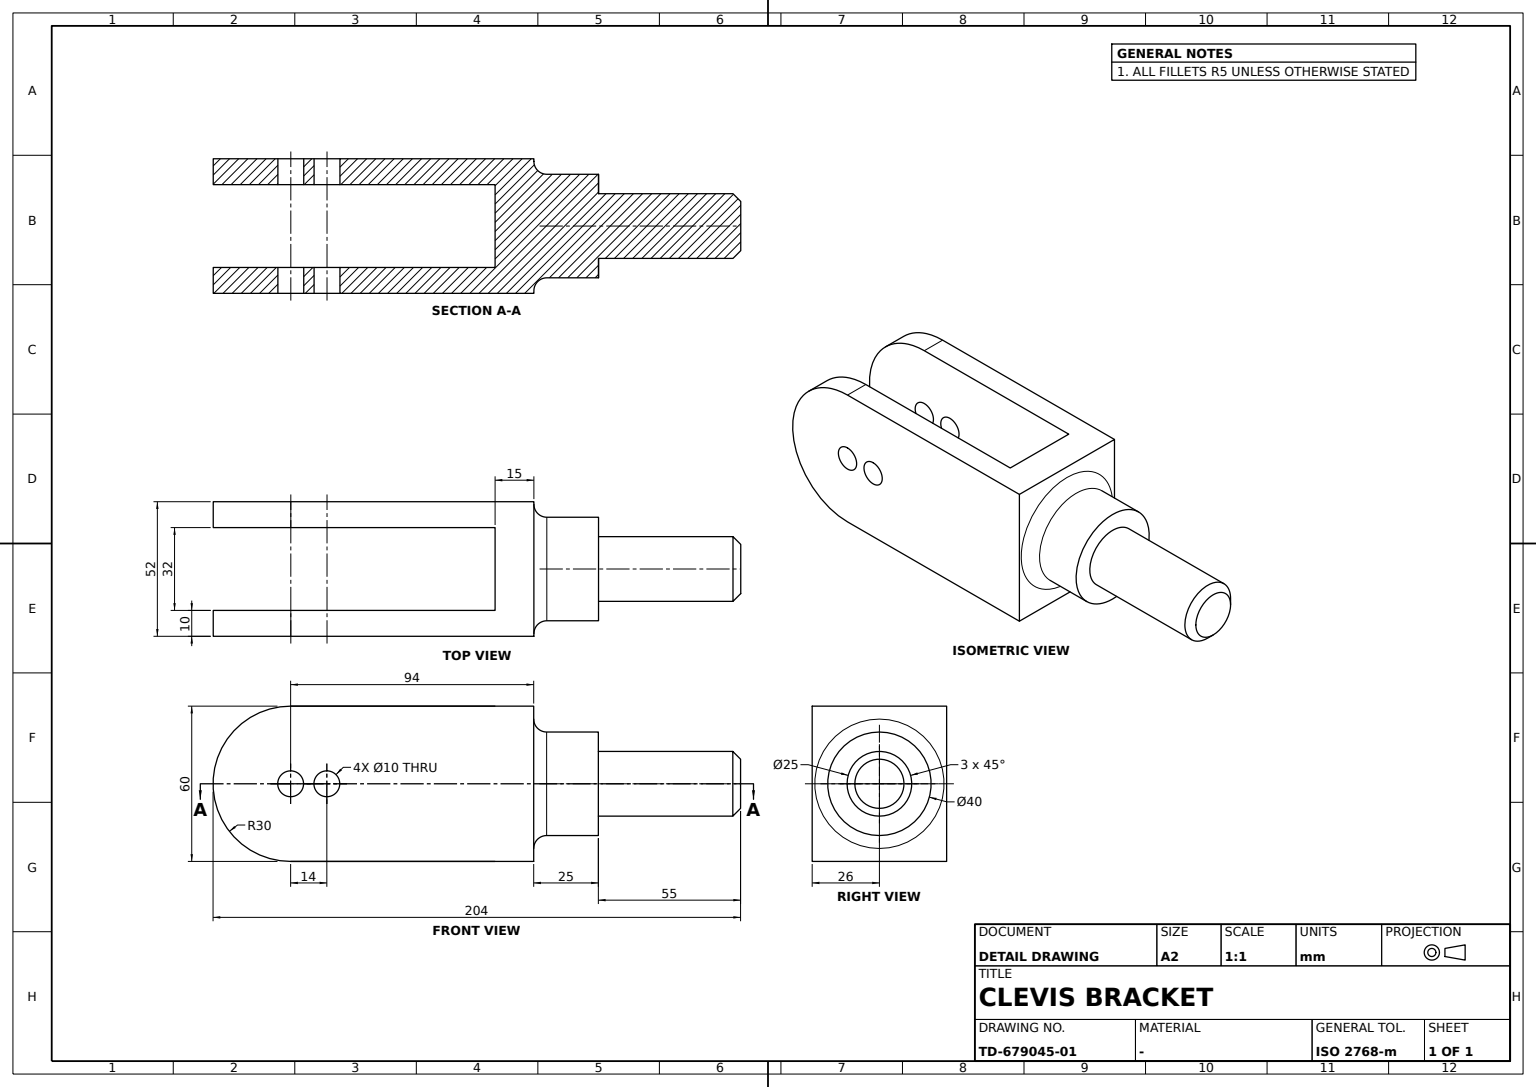
ISO-10303-21;
HEADER;
FILE_DESCRIPTION((''),'2;1');
FILE_NAME('','',(''),(''),'','','');
FILE_SCHEMA(('AUTOMOTIVE_DESIGN'));
ENDSEC;
DATA;
#1=APPLICATION_CONTEXT('');
#2=PRODUCT_CONTEXT('',#1,'mechanical');
#3=PRODUCT('','','',(#2));
#4=PRODUCT_DEFINITION_FORMATION('','',#3);
#5=PRODUCT_DEFINITION_CONTEXT('',#1,'design');
#6=PRODUCT_DEFINITION('','',#4,#5);
#7=PRODUCT_DEFINITION_SHAPE('','',#6);
#8=(LENGTH_UNIT()NAMED_UNIT(*)SI_UNIT(.MILLI.,.METRE.));
#9=(NAMED_UNIT(*)PLANE_ANGLE_UNIT()SI_UNIT($,.RADIAN.));
#10=(NAMED_UNIT(*)SI_UNIT($,.STERADIAN.)SOLID_ANGLE_UNIT());
#11=UNCERTAINTY_MEASURE_WITH_UNIT(LENGTH_MEASURE(0.005),#8,'distance_accuracy_value','');
#12=(GEOMETRIC_REPRESENTATION_CONTEXT(3)GLOBAL_UNCERTAINTY_ASSIGNED_CONTEXT((#11))GLOBAL_UNIT_ASSIGNED_CONTEXT((#8,#9,#10))REPRESENTATION_CONTEXT('',''));
#13=CARTESIAN_POINT('',(-94.,10.,5.));
#14=VERTEX_POINT('',#13);
#15=CARTESIAN_POINT('',(-94.,10.,0.));
#16=DIRECTION('',(0.,1.,0.));
#17=DIRECTION('',(0.,0.,1.));
#18=AXIS2_PLACEMENT_3D('',#15,#16,#17);
#19=CIRCLE('',#18,5.);
#20=EDGE_CURVE('',#14,#14,#19,.T.);
#21=ORIENTED_EDGE('',*,*,#20,.T.);
#22=EDGE_LOOP('',(#21));
#23=FACE_BOUND('',#22,.T.);
#24=CARTESIAN_POINT('',(-94.,0.,5.));
#25=VERTEX_POINT('',#24);
#26=CARTESIAN_POINT('',(-94.,0.,0.));
#27=AXIS2_PLACEMENT_3D('',#26,#16,#17);
#28=CIRCLE('',#27,5.);
#29=EDGE_CURVE('',#25,#25,#28,.T.);
#30=ORIENTED_EDGE('',*,*,#29,.F.);
#31=EDGE_LOOP('',(#30));
#32=FACE_BOUND('',#31,.T.);
#33=CARTESIAN_POINT('',(-94.,5.,0.));
#34=DIRECTION('',(-1.,0.,0.));
#35=AXIS2_PLACEMENT_3D('',#33,#16,#34);
#36=CYLINDRICAL_SURFACE('',#35,5.);
#37=ADVANCED_FACE('',(#23,#32),#36,.F.);
#38=CARTESIAN_POINT('',(-15.,10.,30.));
#39=VERTEX_POINT('',#38);
#40=CARTESIAN_POINT('',(-15.,10.,-30.));
#41=VERTEX_POINT('',#40);
#42=CARTESIAN_POINT('',(-15.,10.,0.));
#43=DIRECTION('',(0.,0.,-1.));
#44=VECTOR('',#43,1000.);
#45=LINE('',#42,#44);
#46=EDGE_CURVE('',#39,#41,#45,.T.);
#47=ORIENTED_EDGE('',*,*,#46,.F.);
#48=CARTESIAN_POINT('',(-15.,42.,30.));
#49=VERTEX_POINT('',#48);
#50=VECTOR('',#16,1000.);
#51=LINE('',#38,#50);
#52=EDGE_CURVE('',#39,#49,#51,.T.);
#53=ORIENTED_EDGE('',*,*,#52,.T.);
#54=CARTESIAN_POINT('',(-15.,42.,-30.));
#55=VERTEX_POINT('',#54);
#56=CARTESIAN_POINT('',(-15.,42.,0.));
#57=LINE('',#56,#44);
#58=EDGE_CURVE('',#49,#55,#57,.T.);
#59=ORIENTED_EDGE('',*,*,#58,.T.);
#60=CARTESIAN_POINT('',(-15.,0.,-30.));
#61=LINE('',#60,#50);
#62=EDGE_CURVE('',#41,#55,#61,.T.);
#63=ORIENTED_EDGE('',*,*,#62,.F.);
#64=EDGE_LOOP('',(#47,#53,#59,#63));
#65=FACE_BOUND('',#64,.T.);
#66=DIRECTION('',(1.,0.,0.));
#67=AXIS2_PLACEMENT_3D('',#38,#66,#43);
#68=PLANE('',#67);
#69=ADVANCED_FACE('',(#65),#68,.F.);
#70=CARTESIAN_POINT('',(0.,26.,25.));
#71=VERTEX_POINT('',#70);
#72=CARTESIAN_POINT('',(0.,26.,0.));
#73=AXIS2_PLACEMENT_3D('',#72,#34,#17);
#74=CIRCLE('',#73,25.);
#75=EDGE_CURVE('',#71,#71,#74,.T.);
#76=ORIENTED_EDGE('',*,*,#75,.F.);
#77=EDGE_LOOP('',(#76));
#78=FACE_BOUND('',#77,.T.);
#79=CARTESIAN_POINT('',(5.,26.,-20.));
#80=VERTEX_POINT('',#79);
#81=CARTESIAN_POINT('',(5.,26.,0.));
#82=AXIS2_PLACEMENT_3D('',#81,#66,#43);
#83=CIRCLE('',#82,20.);
#84=EDGE_CURVE('',#80,#80,#83,.F.);
#85=ORIENTED_EDGE('',*,*,#84,.T.);
#86=EDGE_LOOP('',(#85));
#87=FACE_BOUND('',#86,.T.);
#88=DIRECTION('',(0.,-0.5,-0.866025404));
#89=AXIS2_PLACEMENT_3D('',#81,#34,#88);
#90=TOROIDAL_SURFACE('',#89,25.,5.);
#91=ADVANCED_FACE('',(#78,#87),#90,.F.);
#92=CARTESIAN_POINT('',(-80.,42.,5.));
#93=VERTEX_POINT('',#92);
#94=CARTESIAN_POINT('',(-80.,42.,0.));
#95=AXIS2_PLACEMENT_3D('',#94,#16,#17);
#96=CIRCLE('',#95,5.);
#97=EDGE_CURVE('',#93,#93,#96,.T.);
#98=ORIENTED_EDGE('',*,*,#97,.F.);
#99=EDGE_LOOP('',(#98));
#100=FACE_BOUND('',#99,.T.);
#101=CARTESIAN_POINT('',(-80.,52.,5.));
#102=VERTEX_POINT('',#101);
#103=CARTESIAN_POINT('',(-80.,52.,0.));
#104=AXIS2_PLACEMENT_3D('',#103,#16,#17);
#105=CIRCLE('',#104,5.);
#106=EDGE_CURVE('',#102,#102,#105,.T.);
#107=ORIENTED_EDGE('',*,*,#106,.T.);
#108=EDGE_LOOP('',(#107));
#109=FACE_BOUND('',#108,.T.);
#110=CARTESIAN_POINT('',(-80.,5.,0.));
#111=AXIS2_PLACEMENT_3D('',#110,#16,#34);
#112=CYLINDRICAL_SURFACE('',#111,5.);
#113=ADVANCED_FACE('',(#100,#109),#112,.F.);
#114=ORIENTED_EDGE('',*,*,#52,.F.);
#115=CARTESIAN_POINT('',(-94.,10.,30.));
#116=VERTEX_POINT('',#115);
#117=CARTESIAN_POINT('',(0.,10.,30.));
#118=VECTOR('',#34,1000.);
#119=LINE('',#117,#118);
#120=EDGE_CURVE('',#39,#116,#119,.T.);
#121=ORIENTED_EDGE('',*,*,#120,.T.);
#122=CARTESIAN_POINT('',(-94.,0.,30.));
#123=VERTEX_POINT('',#122);
#124=CARTESIAN_POINT('',(-94.,5.,30.));
#125=LINE('',#124,#50);
#126=EDGE_CURVE('',#123,#116,#125,.T.);
#127=ORIENTED_EDGE('',*,*,#126,.F.);
#128=CARTESIAN_POINT('',(0.,0.,30.));
#129=VERTEX_POINT('',#128);
#130=LINE('',#128,#118);
#131=EDGE_CURVE('',#129,#123,#130,.T.);
#132=ORIENTED_EDGE('',*,*,#131,.F.);
#133=CARTESIAN_POINT('',(0.,52.,30.));
#134=VERTEX_POINT('',#133);
#135=LINE('',#128,#50);
#136=EDGE_CURVE('',#129,#134,#135,.T.);
#137=ORIENTED_EDGE('',*,*,#136,.T.);
#138=CARTESIAN_POINT('',(-94.,52.,30.));
#139=VERTEX_POINT('',#138);
#140=LINE('',#133,#118);
#141=EDGE_CURVE('',#134,#139,#140,.T.);
#142=ORIENTED_EDGE('',*,*,#141,.T.);
#143=CARTESIAN_POINT('',(-94.,42.,30.));
#144=VERTEX_POINT('',#143);
#145=EDGE_CURVE('',#144,#139,#125,.T.);
#146=ORIENTED_EDGE('',*,*,#145,.F.);
#147=CARTESIAN_POINT('',(0.,42.,30.));
#148=LINE('',#147,#118);
#149=EDGE_CURVE('',#49,#144,#148,.T.);
#150=ORIENTED_EDGE('',*,*,#149,.F.);
#151=EDGE_LOOP('',(#114,#121,#127,#132,#137,#142,#146,#150));
#152=FACE_BOUND('',#151,.T.);
#153=AXIS2_PLACEMENT_3D('',#128,#43,#34);
#154=PLANE('',#153);
#155=ADVANCED_FACE('',(#152),#154,.F.);
#156=CARTESIAN_POINT('',(25.,26.,-12.5));
#157=VERTEX_POINT('',#156);
#158=CARTESIAN_POINT('',(25.,26.,0.));
#159=AXIS2_PLACEMENT_3D('',#158,#66,#43);
#160=CIRCLE('',#159,12.5);
#161=EDGE_CURVE('',#157,#157,#160,.T.);
#162=ORIENTED_EDGE('',*,*,#161,.F.);
#163=EDGE_LOOP('',(#162));
#164=FACE_BOUND('',#163,.T.);
#165=CARTESIAN_POINT('',(25.,26.,-20.));
#166=VERTEX_POINT('',#165);
#167=CIRCLE('',#159,20.);
#168=EDGE_CURVE('',#166,#166,#167,.T.);
#169=ORIENTED_EDGE('',*,*,#168,.T.);
#170=EDGE_LOOP('',(#169));
#171=FACE_BOUND('',#170,.T.);
#172=CARTESIAN_POINT('',(25.,0.,0.));
#173=AXIS2_PLACEMENT_3D('',#172,#66,#16);
#174=PLANE('',#173);
#175=ADVANCED_FACE('',(#164,#171),#174,.T.);
#176=CARTESIAN_POINT('',(-80.,10.,5.));
#177=VERTEX_POINT('',#176);
#178=CARTESIAN_POINT('',(-80.,10.,0.));
#179=AXIS2_PLACEMENT_3D('',#178,#16,#17);
#180=CIRCLE('',#179,5.);
#181=EDGE_CURVE('',#177,#177,#180,.T.);
#182=ORIENTED_EDGE('',*,*,#181,.F.);
#183=EDGE_LOOP('',(#182));
#184=FACE_BOUND('',#183,.T.);
#185=CARTESIAN_POINT('',(-94.,10.,-30.));
#186=VERTEX_POINT('',#185);
#187=CIRCLE('',#18,30.);
#188=EDGE_CURVE('',#186,#116,#187,.T.);
#189=ORIENTED_EDGE('',*,*,#188,.T.);
#190=ORIENTED_EDGE('',*,*,#120,.F.);
#191=ORIENTED_EDGE('',*,*,#46,.T.);
#192=CARTESIAN_POINT('',(0.,10.,-30.));
#193=VECTOR('',#66,1000.);
#194=LINE('',#192,#193);
#195=EDGE_CURVE('',#186,#41,#194,.T.);
#196=ORIENTED_EDGE('',*,*,#195,.F.);
#197=EDGE_LOOP('',(#189,#190,#191,#196));
#198=FACE_BOUND('',#197,.T.);
#199=ORIENTED_EDGE('',*,*,#20,.F.);
#200=EDGE_LOOP('',(#199));
#201=FACE_BOUND('',#200,.T.);
#202=CARTESIAN_POINT('',(0.,10.,0.));
#203=AXIS2_PLACEMENT_3D('',#202,#16,#34);
#204=PLANE('',#203);
#205=ADVANCED_FACE('',(#184,#198,#201),#204,.T.);
#206=ORIENTED_EDGE('',*,*,#75,.T.);
#207=EDGE_LOOP('',(#206));
#208=FACE_BOUND('',#207,.T.);
#209=CARTESIAN_POINT('',(0.,0.,-30.));
#210=VERTEX_POINT('',#209);
#211=CARTESIAN_POINT('',(0.,0.,0.));
#212=VECTOR('',#17,1000.);
#213=LINE('',#211,#212);
#214=EDGE_CURVE('',#210,#129,#213,.T.);
#215=ORIENTED_EDGE('',*,*,#214,.F.);
#216=CARTESIAN_POINT('',(0.,52.,-30.));
#217=VERTEX_POINT('',#216);
#218=LINE('',#209,#50);
#219=EDGE_CURVE('',#210,#217,#218,.T.);
#220=ORIENTED_EDGE('',*,*,#219,.T.);
#221=LINE('',#216,#44);
#222=EDGE_CURVE('',#134,#217,#221,.T.);
#223=ORIENTED_EDGE('',*,*,#222,.F.);
#224=ORIENTED_EDGE('',*,*,#136,.F.);
#225=EDGE_LOOP('',(#215,#220,#223,#224));
#226=FACE_BOUND('',#225,.T.);
#227=AXIS2_PLACEMENT_3D('',#209,#34,#17);
#228=PLANE('',#227);
#229=ADVANCED_FACE('',(#208,#226),#228,.F.);
#230=ORIENTED_EDGE('',*,*,#29,.T.);
#231=EDGE_LOOP('',(#230));
#232=FACE_BOUND('',#231,.T.);
#233=CARTESIAN_POINT('',(-80.,0.,5.));
#234=VERTEX_POINT('',#233);
#235=CARTESIAN_POINT('',(-80.,0.,0.));
#236=AXIS2_PLACEMENT_3D('',#235,#16,#17);
#237=CIRCLE('',#236,5.);
#238=EDGE_CURVE('',#234,#234,#237,.T.);
#239=ORIENTED_EDGE('',*,*,#238,.T.);
#240=EDGE_LOOP('',(#239));
#241=FACE_BOUND('',#240,.T.);
#242=ORIENTED_EDGE('',*,*,#131,.T.);
#243=CARTESIAN_POINT('',(-94.,0.,-30.));
#244=VERTEX_POINT('',#243);
#245=CIRCLE('',#27,30.);
#246=EDGE_CURVE('',#244,#123,#245,.T.);
#247=ORIENTED_EDGE('',*,*,#246,.F.);
#248=LINE('',#209,#193);
#249=EDGE_CURVE('',#244,#210,#248,.T.);
#250=ORIENTED_EDGE('',*,*,#249,.T.);
#251=ORIENTED_EDGE('',*,*,#214,.T.);
#252=EDGE_LOOP('',(#242,#247,#250,#251));
#253=FACE_BOUND('',#252,.T.);
#254=AXIS2_PLACEMENT_3D('',#211,#16,#34);
#255=PLANE('',#254);
#256=ADVANCED_FACE('',(#232,#241,#253),#255,.F.);
#257=ORIENTED_EDGE('',*,*,#222,.T.);
#258=CARTESIAN_POINT('',(-94.,52.,-30.));
#259=VERTEX_POINT('',#258);
#260=LINE('',#216,#193);
#261=EDGE_CURVE('',#259,#217,#260,.T.);
#262=ORIENTED_EDGE('',*,*,#261,.F.);
#263=CARTESIAN_POINT('',(-94.,52.,0.));
#264=AXIS2_PLACEMENT_3D('',#263,#16,#17);
#265=CIRCLE('',#264,30.);
#266=EDGE_CURVE('',#259,#139,#265,.T.);
#267=ORIENTED_EDGE('',*,*,#266,.T.);
#268=ORIENTED_EDGE('',*,*,#141,.F.);
#269=EDGE_LOOP('',(#257,#262,#267,#268));
#270=FACE_BOUND('',#269,.T.);
#271=ORIENTED_EDGE('',*,*,#106,.F.);
#272=EDGE_LOOP('',(#271));
#273=FACE_BOUND('',#272,.T.);
#274=CARTESIAN_POINT('',(-94.,52.,5.));
#275=VERTEX_POINT('',#274);
#276=CIRCLE('',#264,5.);
#277=EDGE_CURVE('',#275,#275,#276,.T.);
#278=ORIENTED_EDGE('',*,*,#277,.F.);
#279=EDGE_LOOP('',(#278));
#280=FACE_BOUND('',#279,.T.);
#281=CARTESIAN_POINT('',(0.,52.,0.));
#282=AXIS2_PLACEMENT_3D('',#281,#16,#34);
#283=PLANE('',#282);
#284=ADVANCED_FACE('',(#270,#273,#280),#283,.T.);
#285=CARTESIAN_POINT('',(-94.,42.,5.));
#286=VERTEX_POINT('',#285);
#287=CARTESIAN_POINT('',(-94.,42.,0.));
#288=AXIS2_PLACEMENT_3D('',#287,#16,#17);
#289=CIRCLE('',#288,5.);
#290=EDGE_CURVE('',#286,#286,#289,.T.);
#291=ORIENTED_EDGE('',*,*,#290,.F.);
#292=EDGE_LOOP('',(#291));
#293=FACE_BOUND('',#292,.T.);
#294=ORIENTED_EDGE('',*,*,#277,.T.);
#295=EDGE_LOOP('',(#294));
#296=FACE_BOUND('',#295,.T.);
#297=ADVANCED_FACE('',(#293,#296),#36,.F.);
#298=CARTESIAN_POINT('',(80.,26.,-9.5));
#299=VERTEX_POINT('',#298);
#300=CARTESIAN_POINT('',(80.,26.,0.));
#301=AXIS2_PLACEMENT_3D('',#300,#66,#43);
#302=CIRCLE('',#301,9.5);
#303=EDGE_CURVE('',#299,#299,#302,.T.);
#304=ORIENTED_EDGE('',*,*,#303,.T.);
#305=EDGE_LOOP('',(#304));
#306=FACE_BOUND('',#305,.T.);
#307=CARTESIAN_POINT('',(80.,0.,0.));
#308=AXIS2_PLACEMENT_3D('',#307,#66,#16);
#309=PLANE('',#308);
#310=ADVANCED_FACE('',(#306),#309,.T.);
#311=CARTESIAN_POINT('',(-94.,42.,-30.));
#312=VERTEX_POINT('',#311);
#313=CIRCLE('',#288,30.);
#314=EDGE_CURVE('',#312,#144,#313,.T.);
#315=ORIENTED_EDGE('',*,*,#314,.F.);
#316=CARTESIAN_POINT('',(0.,42.,-30.));
#317=LINE('',#316,#193);
#318=EDGE_CURVE('',#312,#55,#317,.T.);
#319=ORIENTED_EDGE('',*,*,#318,.T.);
#320=ORIENTED_EDGE('',*,*,#58,.F.);
#321=ORIENTED_EDGE('',*,*,#149,.T.);
#322=EDGE_LOOP('',(#315,#319,#320,#321));
#323=FACE_BOUND('',#322,.T.);
#324=ORIENTED_EDGE('',*,*,#290,.T.);
#325=EDGE_LOOP('',(#324));
#326=FACE_BOUND('',#325,.T.);
#327=ORIENTED_EDGE('',*,*,#97,.T.);
#328=EDGE_LOOP('',(#327));
#329=FACE_BOUND('',#328,.T.);
#330=CARTESIAN_POINT('',(0.,42.,0.));
#331=AXIS2_PLACEMENT_3D('',#330,#16,#34);
#332=PLANE('',#331);
#333=ADVANCED_FACE('',(#323,#326,#329),#332,.F.);
#334=ORIENTED_EDGE('',*,*,#249,.F.);
#335=CARTESIAN_POINT('',(-94.,5.,-30.));
#336=LINE('',#335,#50);
#337=EDGE_CURVE('',#244,#186,#336,.T.);
#338=ORIENTED_EDGE('',*,*,#337,.T.);
#339=ORIENTED_EDGE('',*,*,#195,.T.);
#340=ORIENTED_EDGE('',*,*,#62,.T.);
#341=ORIENTED_EDGE('',*,*,#318,.F.);
#342=EDGE_CURVE('',#312,#259,#336,.T.);
#343=ORIENTED_EDGE('',*,*,#342,.T.);
#344=ORIENTED_EDGE('',*,*,#261,.T.);
#345=ORIENTED_EDGE('',*,*,#219,.F.);
#346=EDGE_LOOP('',(#334,#338,#339,#340,#341,#343,#344,#345));
#347=FACE_BOUND('',#346,.T.);
#348=AXIS2_PLACEMENT_3D('',#243,#17,#66);
#349=PLANE('',#348);
#350=ADVANCED_FACE('',(#347),#349,.F.);
#351=CARTESIAN_POINT('',(77.,13.5,0.));
#352=VERTEX_POINT('',#351);
#353=CARTESIAN_POINT('',(77.,26.,0.));
#354=DIRECTION('',(0.,-1.,0.));
#355=AXIS2_PLACEMENT_3D('',#353,#34,#354);
#356=CIRCLE('',#355,12.5);
#357=EDGE_CURVE('',#352,#352,#356,.F.);
#358=ORIENTED_EDGE('',*,*,#357,.T.);
#359=EDGE_LOOP('',(#358));
#360=FACE_BOUND('',#359,.T.);
#361=ORIENTED_EDGE('',*,*,#303,.F.);
#362=EDGE_LOOP('',(#361));
#363=FACE_BOUND('',#362,.T.);
#364=CARTESIAN_POINT('',(89.5,26.,0.));
#365=AXIS2_PLACEMENT_3D('',#364,#34,#354);
#366=CONICAL_SURFACE('',#365,0.,0.785398163);
#367=ADVANCED_FACE('',(#360,#363),#366,.T.);
#368=ORIENTED_EDGE('',*,*,#238,.F.);
#369=EDGE_LOOP('',(#368));
#370=FACE_BOUND('',#369,.T.);
#371=ORIENTED_EDGE('',*,*,#181,.T.);
#372=EDGE_LOOP('',(#371));
#373=FACE_BOUND('',#372,.T.);
#374=ADVANCED_FACE('',(#370,#373),#112,.F.);
#375=ORIENTED_EDGE('',*,*,#357,.F.);
#376=EDGE_LOOP('',(#375));
#377=FACE_BOUND('',#376,.T.);
#378=ORIENTED_EDGE('',*,*,#161,.T.);
#379=EDGE_LOOP('',(#378));
#380=FACE_BOUND('',#379,.T.);
#381=CARTESIAN_POINT('',(52.5,26.,0.));
#382=AXIS2_PLACEMENT_3D('',#381,#66,#16);
#383=CYLINDRICAL_SURFACE('',#382,12.5);
#384=ADVANCED_FACE('',(#377,#380),#383,.T.);
#385=ORIENTED_EDGE('',*,*,#342,.F.);
#386=ORIENTED_EDGE('',*,*,#314,.T.);
#387=ORIENTED_EDGE('',*,*,#145,.T.);
#388=ORIENTED_EDGE('',*,*,#266,.F.);
#389=EDGE_LOOP('',(#385,#386,#387,#388));
#390=FACE_BOUND('',#389,.T.);
#391=CYLINDRICAL_SURFACE('',#35,30.);
#392=ADVANCED_FACE('',(#390),#391,.T.);
#393=ORIENTED_EDGE('',*,*,#126,.T.);
#394=ORIENTED_EDGE('',*,*,#188,.F.);
#395=ORIENTED_EDGE('',*,*,#337,.F.);
#396=ORIENTED_EDGE('',*,*,#246,.T.);
#397=EDGE_LOOP('',(#393,#394,#395,#396));
#398=FACE_BOUND('',#397,.T.);
#399=ADVANCED_FACE('',(#398),#391,.T.);
#400=ORIENTED_EDGE('',*,*,#168,.F.);
#401=EDGE_LOOP('',(#400));
#402=FACE_BOUND('',#401,.T.);
#403=ORIENTED_EDGE('',*,*,#84,.F.);
#404=EDGE_LOOP('',(#403));
#405=FACE_BOUND('',#404,.T.);
#406=CARTESIAN_POINT('',(12.5,26.,0.));
#407=AXIS2_PLACEMENT_3D('',#406,#66,#16);
#408=CYLINDRICAL_SURFACE('',#407,20.);
#409=ADVANCED_FACE('',(#402,#405),#408,.T.);
#410=CLOSED_SHELL('',(#37,#69,#91,#113,#155,#175,#205,#229,#256,#284,#297,#310,#333,#350,#367,#374,#384,#392,#399,#409));
#411=MANIFOLD_SOLID_BREP('',#410);
#412=ADVANCED_BREP_SHAPE_REPRESENTATION('',(#411),#12);
#413=SHAPE_DEFINITION_REPRESENTATION(#7,#412);
ENDSEC;
END-ISO-10303-21;
